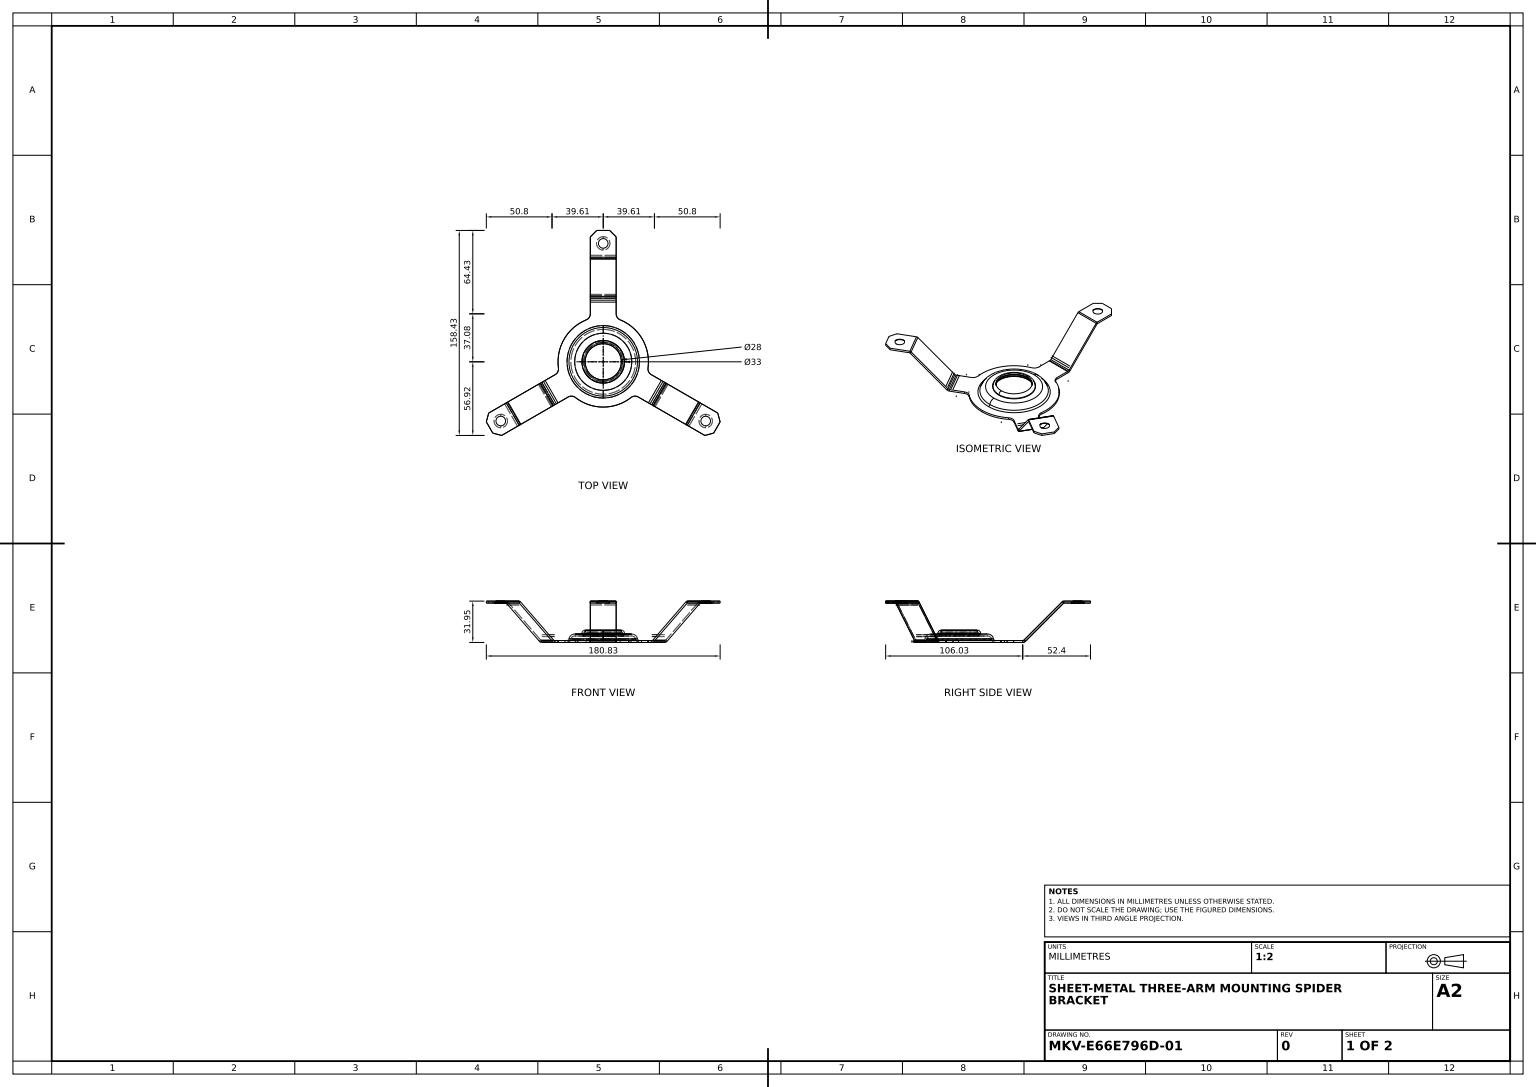
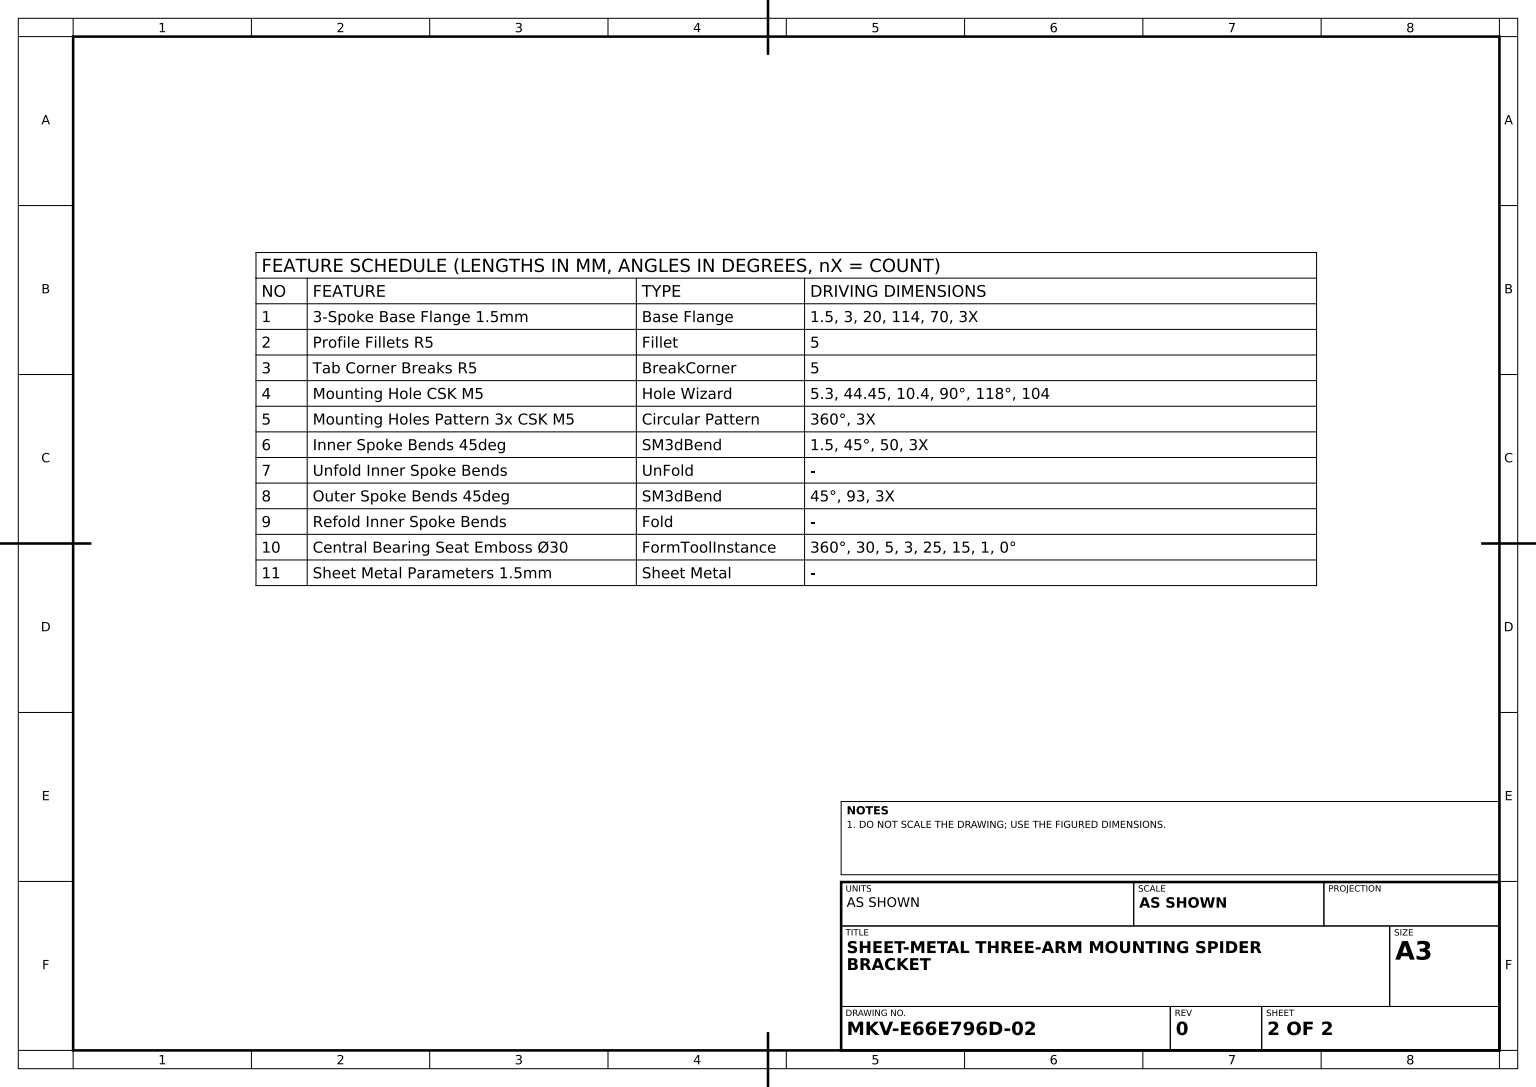
solid
v1 (-10,28.951231,-80.810298)
v2 (-10,30.011891,-79.749638)
e1 v1 v2 LINE
v3 (-10,30.451231,-80.810298)
e2 v3 v2 CIRCLE(AX(P(-10,28.951231,-80.810298),D(1,0,0),D(0,0.707106781,-0.707106781)),1.5)
e3 v1 v3 LINE
face PLANE(AX(P(-10,28.951231,-80.810298),D(1,0,0),D(0,0.707106781,-0.707106781))) rev [e1 -e2 -e3]
v4 (0,6.5,-14)
v5 (0,5.5,-15)
e4 v4 v5 CIRCLE(AX(P(0,5.5,-14),D(-1,0,0),D(0,0,1)),1)
v6 (0,5.5,15)
e5 v5 v6 CIRCLE(AX(P(0,5.5,0),D(0,-1,0),D(0,0,1)),15)
v7 (0,6.5,14)
e6 v7 v6 CIRCLE(AX(P(0,5.5,14),D(1,0,0),D(0,0,-1)),1)
e7 v7 v4 CIRCLE(AX(P(0,6.5,0),D(0,1,0),D(0,0,1)),14)
face TORUS(AX(P(0,5.5,0),D(0,-1,0),D(0,0,1)),14,1) rev [e4 e5 -e6 e7]
v8 (0,3.5,-22.08392)
v9 (0,3.5,22.08392)
e8 v8 v9 CIRCLE(AX(P(0,3.5,0),D(0,1,0),D(0,0,1)),22.08392)
v10 (0,1,25.04196)
e9 v10 v9 CIRCLE(AX(P(0,0.5,22.08392),D(-1,0,0),D(0,0,1)),3)
v11 (0,1,-25.04196)
e10 v10 v11 CIRCLE(AX(P(0,1,0),D(0,-1,0),D(0,0,-1)),25.04196)
e11 v11 v8 CIRCLE(AX(P(0,0.5,-22.08392),D(1,0,0),D(0,0,-1)),3)
face TORUS(AX(P(0,0.5,0),D(0,1,0),D(0,0,-1)),22.08392,3) rev [e8 -e9 e10 e11]
v12 (0,0,-28)
v13 (0,0,28)
e12 v12 v13 CIRCLE(AX(P(0,0,0),D(0,-1,0),D(0,0,-1)),28)
e13 v13 v12 CIRCLE(AX(P(0,0,0),D(0,-1,0),D(0,0,-1)),28)
v14 (10,0,-37.080992)
v15 (10,0,-49.116427)
e14 v14 v15 LINE
v16 (-10,0,-49.116427)
e15 v16 v15 LINE
v17 (-10,0,-37.080992)
e16 v16 v17 LINE
v18 (-13.125,0,-32.445868)
e17 v17 v18 CIRCLE(AX(P(-15,0,-37.080992),D(0,-1,0),D(0,0,1)),5)
v19 (-34.661446,0,4.856351)
e18 v18 v19 CIRCLE(AX(P(0,0,0),D(0,1,0),D(0,0,1)),35)
v20 (-37.113081,0,9.880242)
e19 v19 v20 CIRCLE(AX(P(-39.613081,0,5.550115),D(0,-1,0),D(0,0,1)),5)
v21 (-47.536074,0,15.897959)
e20 v20 v21 LINE
v22 (-37.536074,0,33.218468)
e21 v22 v21 LINE
v23 (-27.113081,0,27.20075)
e22 v22 v23 LINE
v24 (-21.536446,0,27.589518)
e23 v23 v24 CIRCLE(AX(P(-24.613081,0,31.530877),D(0,-1,0),D(0,0,1)),5)
v25 (0,0,35)
e24 v24 v25 CIRCLE(AX(P(0,0,0),D(0,1,0),D(0,0,1)),35)
v26 (21.536446,0,27.589518)
e25 v25 v26 CIRCLE(AX(P(0,0,0),D(0,1,0),D(0,0,1)),35)
v27 (27.113081,0,27.20075)
e26 v26 v27 CIRCLE(AX(P(24.613081,0,31.530877),D(0,-1,0),D(0,0,1)),5)
v28 (37.536074,0,33.218468)
e27 v27 v28 LINE
v29 (47.536074,0,15.897959)
e28 v29 v28 LINE
v30 (37.113081,0,9.880242)
e29 v29 v30 LINE
v31 (34.661446,0,4.856351)
e30 v30 v31 CIRCLE(AX(P(39.613081,0,5.550115),D(0,-1,0),D(0,0,1)),5)
v32 (13.125,0,-32.445868)
e31 v31 v32 CIRCLE(AX(P(0,0,0),D(0,1,0),D(0,0,1)),35)
e32 v32 v14 CIRCLE(AX(P(15,0,-37.080992),D(0,-1,0),D(0,0,1)),5)
face PLANE(AX(P(0,0,0),D(0,1,0),D(0,0,1))) [e12 e13] [e14 -e15 e16 e17 e18 e19 e20 -e21 e22 e23 e24 e25 e26 e27 -e28 e29 e30 e31 e32]
v33 (79.254985,28.951231,40.557887)
v34 (79.254985,28.951231,50.957887)
e33 v33 v34 CIRCLE(AX(P(79.254985,28.951231,45.757887),D(0,-1,0),D(0,0,-1)),5.2)
v35 (79.254985,30.451231,49.457887)
e34 v35 v34 LINE
v36 (79.254985,30.451231,42.057887)
e35 v35 v36 CIRCLE(AX(P(79.254985,30.451231,45.757887),D(0,1,0),D(0,0,1)),3.7)
e36 v36 v33 LINE
face CONE(AX(P(79.254985,28.951231,45.757887),D(0,-1,0),D(0,0,-1)),5.2,0.785398163) rev [e33 -e34 e35 e36]
v37 (0,1.25,26.52098)
e37 v13 v37 CIRCLE(AX(P(0,1.5,28),D(1,0,0),D(0,0,-1)),1.5)
v38 (0,1.25,-26.52098)
e38 v37 v38 CIRCLE(AX(P(0,1.25,0),D(0,-1,0),D(0,0,-1)),26.52098)
e39 v12 v38 CIRCLE(AX(P(0,1.5,-28),D(-1,0,0),D(0,0,1)),1.5)
face TORUS(AX(P(0,1.5,0),D(0,-1,0),D(0,0,1)),28,1.5) rev [-e13 e37 e38 -e39]
v39 (-10,30.451231,-96.515774)
e40 v39 v3 LINE
v40 (10,30.451231,-80.810298)
e41 v3 v40 LINE
v41 (10,30.451231,-96.515774)
e42 v40 v41 LINE
v42 (5,30.451231,-101.515774)
e43 v41 v42 LINE
v43 (-5,30.451231,-101.515774)
e44 v42 v43 LINE
e45 v43 v39 LINE
v44 (0,30.451231,-95.215774)
v45 (0,30.451231,-87.815774)
e46 v44 v45 CIRCLE(AX(P(0,30.451231,-91.515774),D(0,1,0),D(0,0,1)),3.7)
e47 v45 v44 CIRCLE(AX(P(0,30.451231,-91.515774),D(0,1,0),D(0,0,1)),3.7)
face PLANE(AX(P(0,30.451231,12.484226),D(0,1,0),D(0,0,1))) [e40 e41 e42 e43 e44 e45] [-e46 -e47]
e48 v34 v33 CIRCLE(AX(P(79.254985,28.951231,45.757887),D(0,-1,0),D(0,0,-1)),5.2)
e49 v36 v35 CIRCLE(AX(P(79.254985,30.451231,45.757887),D(0,1,0),D(0,0,1)),3.7)
face CONE(AX(P(79.254985,28.951231,45.757887),D(0,-1,0),D(0,0,-1)),5.2,0.785398163) rev [e34 e48 -e36 e49]
v46 (85.415239,30.451231,55.088014)
v47 (90.415239,30.451231,46.42776)
e50 v46 v47 LINE
v48 (85.415239,28.951231,55.088014)
e51 v46 v48 LINE
v49 (90.415239,28.951231,46.42776)
e52 v48 v49 LINE
e53 v49 v47 LINE
face PLANE(AX(P(92.915239,28.951231,42.097633),D(0.866025404,0,0.5),D(0.5,0,-0.866025404))) [-e50 e51 e52 e53]
v50 (0,5,16.5)
v51 (0,5,-16.5)
e54 v50 v51 CIRCLE(AX(P(0,5,0),D(0,1,0),D(0,0,-1)),16.5)
e55 v51 v50 CIRCLE(AX(P(0,5,0),D(0,1,0),D(0,0,-1)),16.5)
v52 (0,5,-22.08392)
v53 (0,5,22.08392)
e56 v52 v53 CIRCLE(AX(P(0,5,0),D(0,1,0),D(0,0,1)),22.08392)
e57 v53 v52 CIRCLE(AX(P(0,5,0),D(0,1,0),D(0,0,1)),22.08392)
face PLANE(AX(P(-25,5,0),D(0,-1,0),D(0,0,1))) rev [-e54 -e55] [e56 e57]
v54 (-37.536074,-1.5,33.218468)
v55 (-27.113081,-1.5,27.20075)
e58 v54 v55 LINE
e59 v55 v23 LINE
e60 v54 v22 LINE
face PLANE(AX(P(-24.047375,-1.5,25.430764),D(0.5,0,0.866025404),D(0.866025404,0,-0.5))) [e58 e59 -e22 -e60]
v56 (10,28.951231,-80.810298)
e61 v40 v56 LINE
v57 (10,28.951231,-96.515774)
e62 v56 v57 LINE
e63 v57 v41 LINE
face PLANE(AX(P(10,28.951231,-21.056794),D(1,0,0),D(0,0,-1))) [-e42 e61 e62 e63]
v58 (27.113081,-1.5,27.20075)
e64 v27 v58 LINE
v59 (37.536074,-1.5,33.218468)
e65 v58 v59 LINE
e66 v28 v59 LINE
face PLANE(AX(P(24.047375,-1.5,25.430764),D(-0.5,0,0.866025404),D(0.866025404,0,0.5))) [e64 e65 -e66 -e27]
v60 (64.983771,30.451231,49.065403)
v61 (78.585112,30.451231,56.918141)
e67 v60 v61 LINE
v62 (64.983771,28.951231,49.065403)
e68 v60 v62 LINE
v63 (78.585112,28.951231,56.918141)
e69 v62 v63 LINE
e70 v63 v61 LINE
face PLANE(AX(P(13.235718,28.951231,19.188651),D(-0.5,0,0.866025404),D(0.866025404,0,0.5))) [-e67 e68 e69 e70]
e71 v9 v8 CIRCLE(AX(P(0,3.5,0),D(0,1,0),D(0,0,1)),22.08392)
e72 v11 v10 CIRCLE(AX(P(0,1,0),D(0,-1,0),D(0,0,-1)),25.04196)
face TORUS(AX(P(0,0.5,0),D(0,1,0),D(0,0,-1)),22.08392,3) rev [e71 -e11 e72 e9]
v64 (34.661446,-1.5,4.856351)
e73 v31 v64 LINE
v65 (13.125,-1.5,-32.445868)
e74 v64 v65 CIRCLE(AX(P(0,-1.5,0),D(0,1,0),D(0,0,1)),35)
e75 v65 v32 LINE
face CYL(AX(P(0,-1.5,0),D(0,1,0),D(0,0,1)),35) [-e31 e73 e74 e75]
v66 (0,-1.5,28)
e76 v66 v10 CIRCLE(AX(P(0,1.5,28),D(1,0,0),D(0,0,-1)),3)
v67 (0,-1.5,-28)
e77 v66 v67 CIRCLE(AX(P(0,-1.5,0),D(0,-1,0),D(0,0,1)),28)
e78 v67 v11 CIRCLE(AX(P(0,1.5,-28),D(-1,0,0),D(0,0,1)),3)
face TORUS(AX(P(0,1.5,0),D(0,-1,0),D(0,0,1)),28,3) [-e10 -e76 e77 e78]
v68 (0,28.951231,-86.315774)
e79 v45 v68 LINE
v69 (0,28.951231,-96.715774)
e80 v68 v69 CIRCLE(AX(P(0,28.951231,-91.515774),D(0,-1,0),D(0,0,-1)),5.2)
e81 v44 v69 LINE
face CONE(AX(P(0,28.951231,-91.515774),D(0,-1,0),D(0,0,-1)),5.2,0.785398163) rev [e46 e79 e80 -e81]
v70 (-38.454632,0.43934,33.748798)
e82 v22 v70 CIRCLE(AX(P(-37.536074,1.5,33.218468),D(-0.5,0,-0.866025404),D(-0.866025404,0,0.5)),1.5)
v71 (-39.373191,-0.62132,34.279128)
e83 v71 v70 LINE
e84 v54 v71 CIRCLE(AX(P(-37.536074,1.5,33.218468),D(-0.5,0,-0.866025404),D(-0.866025404,0,0.5)),3)
face PLANE(AX(P(-37.536074,1.5,33.218468),D(0.5,0,0.866025404),D(0.866025404,0,-0.5))) [e60 e82 -e83 -e84]
v72 (10,-1.5,-49.116427)
e85 v15 v72 LINE
v73 (10,-1.5,-37.080992)
e86 v14 v73 LINE
e87 v73 v72 LINE
face PLANE(AX(P(10,-1.5,-33.54102),D(1,0,0),D(0,0,-1))) [-e85 -e14 e86 e87]
v74 (-64.983771,28.951231,49.065403)
v75 (-64.983771,30.451231,49.065403)
e88 v74 v75 LINE
v76 (-64.065213,30.011891,48.535073)
e89 v74 v76 LINE
e90 v75 v76 CIRCLE(AX(P(-64.983771,28.951231,49.065403),D(-0.5,0,-0.866025404),D(-0.612372436,0.707106781,0.353553391)),1.5)
face PLANE(AX(P(-64.983771,28.951231,49.065403),D(-0.5,0,-0.866025404),D(-0.612372436,0.707106781,0.353553391))) rev [-e88 e89 -e90]
v77 (47.536074,-1.5,15.897959)
e91 v77 v29 LINE
v78 (37.113081,-1.5,9.880242)
e92 v77 v78 LINE
e93 v78 v30 LINE
face PLANE(AX(P(34.047375,-1.5,8.110256),D(0.5,0,-0.866025404),D(-0.866025404,0,-0.5))) [-e91 e92 e93 -e29]
v79 (49.373191,-0.62132,16.95862)
v80 (39.373191,-0.62132,34.279128)
e94 v79 v80 LINE
e95 v80 v59 CIRCLE(AX(P(37.536074,1.5,33.218468),D(0.5,0,-0.866025404),D(-0.866025404,0,-0.5)),3)
e96 v77 v59 LINE
e97 v77 v79 CIRCLE(AX(P(47.536074,1.5,15.897959),D(-0.5,0,0.866025404),D(0.866025404,0,0.5)),3)
face CYL(AX(P(53.336404,1.5,5.851493),D(-0.5,0,0.866025404),D(0.866025404,0,0.5)),3) [e94 e95 -e96 e97]
v81 (-10,-1.5,-49.116427)
e98 v81 v16 LINE
v82 (-10,-1.5,-37.080992)
e99 v81 v82 LINE
e100 v82 v17 LINE
face PLANE(AX(P(-10,-1.5,-33.54102),D(-1,0,0),D(0,0,1))) [-e16 -e98 e99 e100]
v83 (5,28.951231,-101.515774)
v84 (-5,28.951231,-101.515774)
e101 v83 v84 LINE
e102 v84 v43 LINE
e103 v42 v83 LINE
face PLANE(AX(P(-10,28.951231,-101.515774),D(0,0,-1),D(-1,0,0))) [e101 e102 -e44 e103]
v85 (-90.415239,30.451231,46.42776)
v86 (-90.415239,28.951231,46.42776)
e104 v85 v86 LINE
v87 (-88.585112,30.451231,39.597633)
e105 v87 v85 LINE
v88 (-88.585112,28.951231,39.597633)
e106 v88 v87 LINE
e107 v86 v88 LINE
face PLANE(AX(P(-88.585112,28.951231,39.597633),D(0.965925826,0,0.258819045),D(0,1,0))) rev [-e104 -e105 -e106 -e107]
v89 (48.454632,0.43934,16.42829)
e108 v29 v89 CIRCLE(AX(P(47.536074,1.5,15.897959),D(-0.5,0,0.866025404),D(0.866025404,0,0.5)),1.5)
v90 (38.454632,0.43934,33.748798)
e109 v90 v28 CIRCLE(AX(P(37.536074,1.5,33.218468),D(0.5,0,-0.866025404),D(0.866025404,0,0.5)),1.5)
e110 v89 v90 LINE
face CYL(AX(P(53.336404,1.5,5.851493),D(-0.5,0,0.866025404),D(0.866025404,0,0.5)),1.5) rev [-e108 e28 -e109 -e110]
v91 (74.983771,28.951231,31.744895)
e111 v91 v79 LINE
e112 v79 v89 LINE
v92 (74.065213,30.011891,31.214565)
e113 v92 v89 LINE
e114 v91 v92 LINE
face PLANE(AX(P(38.753089,-12.884357,10.827101),D(0.5,0,-0.866025404),D(-0.612372436,-0.707106781,-0.353553391))) [e111 e112 -e113 -e114]
v93 (-74.983771,30.451231,31.744895)
e115 v75 v93 LINE
v94 (-74.065213,30.011891,31.214565)
e116 v76 v94 LINE
e117 v93 v94 CIRCLE(AX(P(-74.983771,28.951231,31.744895),D(-0.5,0,-0.866025404),D(-0.612372436,0.707106781,0.353553391)),1.5)
face CYL(AX(P(-74.983771,28.951231,31.744895),D(-0.5,0,-0.866025404),D(-0.612372436,0.707106781,0.353553391)),1.5) [-e115 e90 e116 -e117]
e118 v4 v7 CIRCLE(AX(P(0,6.5,0),D(0,1,0),D(0,0,1)),14)
v95 (0,8,-14)
e119 v95 v4 LINE
v96 (0,8,14)
e120 v95 v96 CIRCLE(AX(P(0,8,0),D(0,1,0),D(0,0,-1)),14)
e121 v96 v7 LINE
face CYL(AX(P(0,5.5,0),D(0,-1,0),D(0,0,-1)),14) rev [-e118 -e119 e120 e121]
e122 v67 v66 CIRCLE(AX(P(0,-1.5,0),D(0,-1,0),D(0,0,1)),28)
face TORUS(AX(P(0,1.5,0),D(0,-1,0),D(0,0,1)),28,3) [-e78 e122 e76 -e72]
e123 v38 v37 CIRCLE(AX(P(0,1.25,0),D(0,-1,0),D(0,0,-1)),26.52098)
face TORUS(AX(P(0,1.5,0),D(0,-1,0),D(0,0,1)),28,1.5) rev [-e37 -e12 e39 e123]
v97 (10,30.011891,-79.749638)
e124 v40 v97 CIRCLE(AX(P(10,28.951231,-80.810298),D(1,0,0),D(0,0.707106781,-0.707106781)),1.5)
e125 v97 v56 LINE
face PLANE(AX(P(10,28.951231,-80.810298),D(-1,0,0),D(0,-0.707106781,0.707106781))) rev [e124 e125 -e61]
e126 v73 v65 CIRCLE(AX(P(15,-1.5,-37.080992),D(0,1,0),D(0,0,1)),5)
face CYL(AX(P(15,-1.5,-37.080992),D(0,1,0),D(0,0,1)),5) rev [-e126 -e86 -e32 -e75]
face PLANE(AX(P(47.536074,1.5,15.897959),D(0.5,0,-0.866025404),D(-0.866025404,0,-0.5))) [-e97 e91 e108 -e112]
v98 (-49.373191,-0.62132,16.95862)
v99 (-74.983771,28.951231,31.744895)
e127 v98 v99 LINE
e128 v94 v99 LINE
v100 (-48.454632,0.43934,16.42829)
e129 v100 v94 LINE
e130 v100 v98 LINE
face PLANE(AX(P(-38.753089,-12.884357,10.827101),D(-0.5,0,-0.866025404),D(-0.612372436,0.707106781,0.353553391))) [e127 -e128 -e129 e130]
v101 (-79.254985,30.451231,49.457887)
v102 (-79.254985,30.451231,42.057887)
e131 v101 v102 CIRCLE(AX(P(-79.254985,30.451231,45.757887),D(0,1,0),D(0,0,1)),3.7)
v103 (-79.254985,28.951231,40.557887)
e132 v102 v103 LINE
v104 (-79.254985,28.951231,50.957887)
e133 v103 v104 CIRCLE(AX(P(-79.254985,28.951231,45.757887),D(0,-1,0),D(0,0,-1)),5.2)
e134 v101 v104 LINE
face CONE(AX(P(-79.254985,28.951231,45.757887),D(0,-1,0),D(0,0,-1)),5.2,0.785398163) rev [e131 e132 e133 -e134]
v105 (-85.415239,30.451231,55.088014)
v106 (-78.585112,30.451231,56.918141)
e135 v105 v106 LINE
e136 v106 v75 LINE
e137 v93 v87 LINE
e138 v85 v105 LINE
e139 v102 v101 CIRCLE(AX(P(-79.254985,30.451231,45.757887),D(0,1,0),D(0,0,1)),3.7)
face PLANE(AX(P(10.811657,30.451231,-6.242113),D(0,1,0),D(0,0,1))) [e135 e136 e115 e137 e105 e138] [-e131 -e139]
v107 (74.983771,30.451231,31.744895)
e140 v91 v107 LINE
v108 (88.585112,30.451231,39.597633)
e141 v108 v107 LINE
v109 (88.585112,28.951231,39.597633)
e142 v108 v109 LINE
e143 v109 v91 LINE
face PLANE(AX(P(23.235718,28.951231,1.868143),D(0.5,0,-0.866025404),D(-0.866025404,0,-0.5))) [e140 -e141 e142 e143]
e144 v99 v88 LINE
e145 v93 v99 LINE
face PLANE(AX(P(-23.235718,28.951231,1.868143),D(-0.5,0,-0.866025404),D(-0.866025404,0,0.5))) [e144 e106 -e137 e145]
v110 (0,5.5,-16.5)
e146 v95 v110 CIRCLE(AX(P(0,5.5,-14),D(-1,0,0),D(0,0,1)),2.5)
e147 v96 v95 CIRCLE(AX(P(0,8,0),D(0,1,0),D(0,0,-1)),14)
v111 (0,5.5,16.5)
e148 v96 v111 CIRCLE(AX(P(0,5.5,14),D(1,0,0),D(0,0,-1)),2.5)
e149 v110 v111 CIRCLE(AX(P(0,5.5,0),D(0,-1,0),D(0,0,1)),16.5)
face TORUS(AX(P(0,5.5,0),D(0,-1,0),D(0,0,1)),14,2.5) [-e146 -e147 e148 -e149]
v112 (21.536446,-1.5,27.589518)
e150 v58 v112 CIRCLE(AX(P(24.613081,-1.5,31.530877),D(0,1,0),D(0,0,1)),5)
e151 v112 v26 LINE
face CYL(AX(P(24.613081,-1.5,31.530877),D(0,1,0),D(0,0,1)),5) rev [-e150 -e64 -e26 -e151]
v113 (-37.113081,-1.5,9.880242)
e152 v20 v113 LINE
v114 (-47.536074,-1.5,15.897959)
e153 v113 v114 LINE
e154 v21 v114 LINE
face PLANE(AX(P(-34.047375,-1.5,8.110256),D(-0.5,0,-0.866025404),D(-0.866025404,0,0.5))) [-e20 e152 e153 -e154]
face PLANE(AX(P(-74.983771,28.951231,31.744895),D(0.5,0,0.866025404),D(0.612372436,-0.707106781,-0.353553391))) rev [-e145 e117 e128]
e155 v48 v63 LINE
e156 v61 v46 LINE
face PLANE(AX(P(78.585112,28.951231,56.918141),D(-0.258819045,0,-0.965925826),D(0,1,0))) rev [-e70 -e155 -e51 -e156]
e157 v98 v114 CIRCLE(AX(P(-47.536074,1.5,15.897959),D(0.5,0,0.866025404),D(0.866025404,0,-0.5)),3)
e158 v100 v21 CIRCLE(AX(P(-47.536074,1.5,15.897959),D(0.5,0,0.866025404),D(-0.866025404,0,0.5)),1.5)
face PLANE(AX(P(-47.536074,1.5,15.897959),D(-0.5,0,-0.866025404),D(-0.866025404,0,0.5))) [-e157 -e130 e158 e154]
e159 v47 v108 LINE
e160 v107 v60 LINE
face PLANE(AX(P(-10.811657,30.451231,-6.242113),D(0,1,0),D(0,0,1))) [e67 e156 e50 e159 e141 e160] [-e49 -e35]
v115 (64.065213,30.011891,48.535073)
e161 v92 v115 LINE
e162 v60 v115 CIRCLE(AX(P(64.983771,28.951231,49.065403),D(-0.5,0,0.866025404),D(0.612372436,0.707106781,0.353553391)),1.5)
e163 v107 v92 CIRCLE(AX(P(74.983771,28.951231,31.744895),D(-0.5,0,0.866025404),D(0.612372436,0.707106781,0.353553391)),1.5)
face CYL(AX(P(64.983771,28.951231,49.065403),D(-0.5,0,0.866025404),D(0.612372436,0.707106781,0.353553391)),1.5) [e161 -e162 -e160 e163]
e164 v50 v111 LINE
e165 v51 v110 LINE
face CYL(AX(P(0,6.5,0),D(0,1,0),D(0,0,-1)),16.5) [e149 -e164 e54 e165]
e166 v111 v110 CIRCLE(AX(P(0,5.5,0),D(0,-1,0),D(0,0,1)),16.5)
face CYL(AX(P(0,6.5,0),D(0,1,0),D(0,0,-1)),16.5) [e164 e166 -e165 e55]
v116 (-78.585112,28.951231,56.918141)
e167 v106 v116 LINE
e168 v116 v74 LINE
face PLANE(AX(P(-13.235718,28.951231,19.188651),D(0.5,0,0.866025404),D(0.866025404,0,-0.5))) [e167 e168 e88 -e136]
v117 (-10,28.951231,-96.515774)
e169 v117 v1 LINE
e170 v39 v117 LINE
face PLANE(AX(P(-10,28.951231,-21.056794),D(-1,0,0),D(0,0,1))) [e169 e3 -e40 e170]
v118 (-21.536446,-1.5,27.589518)
e171 v24 v118 LINE
v119 (0,-1.5,35)
e172 v118 v119 CIRCLE(AX(P(0,-1.5,0),D(0,1,0),D(0,0,1)),35)
e173 v119 v25 LINE
face CYL(AX(P(0,-1.5,0),D(0,1,0),D(0,0,1)),35) [-e24 e171 e172 e173]
e174 v2 v97 LINE
face CYL(AX(P(10,28.951231,-80.810298),D(1,0,0),D(0,0.707106781,-0.707106781)),1.5) [e2 e174 -e124 -e41]
v120 (0,4.5,15)
e175 v120 v6 LINE
v121 (0,4.5,-15)
e176 v121 v5 LINE
e177 v120 v121 CIRCLE(AX(P(0,4.5,0),D(0,1,0),D(0,0,1)),15)
face CYL(AX(P(0,6.5,0),D(0,1,0),D(0,0,-1)),15) rev [e175 -e5 -e176 -e177]
v122 (-10,0.43934,-50.177087)
v123 (10,0.43934,-50.177087)
e178 v122 v123 LINE
e179 v123 v97 LINE
e180 v2 v122 LINE
face PLANE(AX(P(0,-35.54078,-14.196968),D(0,0.707106781,0.707106781),D(0,-0.707106781,0.707106781))) [e178 e179 -e174 e180]
face PLANE(AX(P(74.983771,28.951231,31.744895),D(-0.5,0,0.866025404),D(0.612372436,0.707106781,0.353553391))) rev [-e163 -e140 e114]
v124 (-10,-0.62132,-51.237747)
e181 v1 v124 LINE
e182 v1 v56 LINE
v125 (10,-0.62132,-51.237747)
e183 v125 v56 LINE
e184 v124 v125 LINE
face PLANE(AX(P(0,-36.60144,-15.257628),D(0,0.707106781,0.707106781),D(0,-0.707106781,0.707106781))) rev [-e181 e182 -e183 -e184]
v126 (0,3.5,16)
v127 (0,3.5,-16)
e185 v126 v127 CIRCLE(AX(P(0,3.5,0),D(0,-1,0),D(0,0,1)),16)
e186 v127 v126 CIRCLE(AX(P(0,3.5,0),D(0,-1,0),D(0,0,1)),16)
face PLANE(AX(P(-25,3.5,0),D(0,-1,0),D(0,0,1))) [-e71 -e8] [-e185 -e186]
e187 v38 v52 CIRCLE(AX(P(0,0.5,-22.08392),D(1,0,0),D(0,0,-1)),4.5)
e188 v37 v53 CIRCLE(AX(P(0,0.5,22.08392),D(-1,0,0),D(0,0,1)),4.5)
face TORUS(AX(P(0,0.5,0),D(0,1,0),D(0,0,-1)),22.08392,4.5) [-e123 e187 -e57 -e188]
e189 v64 v78 CIRCLE(AX(P(39.613081,-1.5,5.550115),D(0,1,0),D(0,0,1)),5)
face CYL(AX(P(39.613081,-1.5,5.550115),D(0,1,0),D(0,0,1)),5) rev [-e30 -e93 -e189 -e73]
v128 (-34.661446,-1.5,4.856351)
e190 v128 v19 LINE
v129 (-13.125,-1.5,-32.445868)
e191 v18 v129 LINE
e192 v129 v128 CIRCLE(AX(P(0,-1.5,0),D(0,1,0),D(0,0,1)),35)
face CYL(AX(P(0,-1.5,0),D(0,1,0),D(0,0,1)),35) [e190 -e18 e191 e192]
e193 v113 v128 CIRCLE(AX(P(-39.613081,-1.5,5.550115),D(0,1,0),D(0,0,1)),5)
face CYL(AX(P(-39.613081,-1.5,5.550115),D(0,1,0),D(0,0,1)),5) rev [-e152 -e19 -e190 -e193]
e194 v125 v72 CIRCLE(AX(P(10,1.5,-49.116427),D(-1,0,0),D(0,0,1)),3)
e195 v81 v72 LINE
e196 v81 v124 CIRCLE(AX(P(-10,1.5,-49.116427),D(1,0,0),D(0,0,-1)),3)
face CYL(AX(P(-20.133872,1.5,-49.116427),D(1,0,0),D(0,0,-1)),3) [e194 -e195 e196 e184]
v130 (-85.415239,28.951231,55.088014)
e197 v86 v130 LINE
e198 v74 v99 LINE
e199 v116 v130 LINE
e200 v104 v103 CIRCLE(AX(P(-79.254985,28.951231,45.757887),D(0,-1,0),D(0,0,-1)),5.2)
face PLANE(AX(P(10.811657,28.951231,-6.242113),D(0,1,0),D(0,0,1))) rev [-e197 e107 -e144 -e198 -e168 e199] [-e200 -e133]
e201 v90 v80 LINE
face PLANE(AX(P(37.536074,1.5,33.218468),D(-0.5,0,0.866025404),D(0.866025404,0,0.5))) [e109 e66 -e95 -e201]
e202 v123 v125 LINE
face PLANE(AX(P(10,-12.884357,-38.97471),D(1,0,0),D(0,0.707106781,-0.707106781))) [-e125 -e179 e202 e183]
e203 v16 v122 CIRCLE(AX(P(-10,1.5,-49.116427),D(1,0,0),D(0,0,-1)),1.5)
e204 v124 v122 LINE
face PLANE(AX(P(-10,1.5,-49.116427),D(-1,0,0),D(0,0,1))) [e203 -e204 -e196 e98]
e205 v115 v62 LINE
face PLANE(AX(P(64.983771,28.951231,49.065403),D(0.5,0,-0.866025404),D(-0.612372436,-0.707106781,-0.353553391))) rev [e162 e205 -e68]
e206 v70 v100 LINE
face CYL(AX(P(-31.735743,1.5,43.264934),D(-0.5,0,-0.866025404),D(-0.866025404,0,0.5)),1.5) rev [-e158 -e206 -e82 e21]
e207 v118 v55 CIRCLE(AX(P(-24.613081,-1.5,31.530877),D(0,1,0),D(0,0,1)),5)
face CYL(AX(P(-24.613081,-1.5,31.530877),D(0,1,0),D(0,0,1)),5) rev [-e171 -e23 -e59 -e207]
e208 v6 v5 CIRCLE(AX(P(0,5.5,0),D(0,-1,0),D(0,0,1)),15)
face TORUS(AX(P(0,5.5,0),D(0,-1,0),D(0,0,1)),14,1) rev [e118 e6 e208 -e4]
e209 v109 v49 LINE
face PLANE(AX(P(90.415239,28.951231,46.42776),D(-0.965925826,0,0.258819045),D(0,1,0))) rev [-e142 -e159 -e53 -e209]
face CYL(AX(P(0,5.5,0),D(0,-1,0),D(0,0,-1)),14) rev [e119 -e7 -e121 e147]
e210 v123 v15 CIRCLE(AX(P(10,1.5,-49.116427),D(-1,0,0),D(0,0,-1)),1.5)
face PLANE(AX(P(10,1.5,-49.116427),D(1,0,0),D(0,0,-1))) [e210 e85 -e194 -e202]
face PLANE(AX(P(-10,-12.884357,-38.97471),D(-1,0,0),D(0,-0.707106781,0.707106781))) [e204 -e180 -e1 e181]
face CYL(AX(P(-20.133872,1.5,-49.116427),D(1,0,0),D(0,0,-1)),1.5) rev [-e210 -e178 -e203 e15]
e211 v54 v114 LINE
e212 v129 v82 CIRCLE(AX(P(-15,-1.5,-37.080992),D(0,1,0),D(0,0,1)),5)
e213 v119 v112 CIRCLE(AX(P(0,-1.5,0),D(0,1,0),D(0,0,1)),35)
face PLANE(AX(P(0,-1.5,0),D(0,1,0),D(0,0,1))) rev [-e172 e207 -e58 e211 -e153 e193 -e192 e212 -e99 e195 -e87 e126 -e74 e189 -e92 e96 -e65 e150 -e213] [-e77 -e122]
e214 v117 v84 LINE
e215 v83 v57 LINE
e216 v69 v68 CIRCLE(AX(P(0,28.951231,-91.515774),D(0,-1,0),D(0,0,-1)),5.2)
face PLANE(AX(P(0,28.951231,12.484226),D(0,1,0),D(0,0,1))) rev [-e182 -e169 e214 -e101 e215 -e62] [-e216 -e80]
e217 v76 v70 LINE
e218 v74 v71 LINE
face PLANE(AX(P(-28.753089,-12.884357,28.147609),D(0.5,0,0.866025404),D(0.612372436,-0.707106781,-0.353553391))) [-e217 -e89 e218 e83]
face TORUS(AX(P(0,0.5,0),D(0,1,0),D(0,0,-1)),22.08392,4.5) [-e56 -e187 -e38 e188]
e219 v91 v62 LINE
e220 v80 v62 LINE
face PLANE(AX(P(13.213493,-36.60144,7.628814),D(-0.612372436,0.707106781,-0.353553391),D(-0.126826484,0.353553391,0.926776695))) rev [-e94 -e111 e219 -e220]
e221 v130 v105 LINE
face PLANE(AX(P(-85.415239,28.951231,55.088014),D(0.258819045,0,-0.965925826),D(0,1,0))) rev [-e135 -e221 -e199 -e167]
e222 v90 v115 LINE
face PLANE(AX(P(28.753089,-12.884357,28.147609),D(-0.5,0,0.866025404),D(0.612372436,0.707106781,0.353553391))) [-e222 e201 e220 -e205]
e223 v71 v98 LINE
face PLANE(AX(P(-13.213493,-36.60144,7.628814),D(0.612372436,0.707106781,-0.353553391),D(0.126826484,0.353553391,0.926776695))) rev [-e223 -e218 e198 -e127]
face PLANE(AX(P(-5,28.951231,-101.515774),D(0.707106781,0,0.707106781),D(0,1,0))) rev [-e170 -e45 -e102 -e214]
e224 v121 v120 CIRCLE(AX(P(0,4.5,0),D(0,1,0),D(0,0,1)),15)
face CYL(AX(P(0,6.5,0),D(0,1,0),D(0,0,-1)),15) rev [-e175 -e224 e176 -e208]
e225 v126 v120 CIRCLE(AX(P(0,4.5,16),D(1,0,0),D(0,0,-1)),1)
e226 v127 v121 CIRCLE(AX(P(0,4.5,-16),D(-1,0,0),D(0,0,1)),1)
face TORUS(AX(P(0,4.5,0),D(0,-1,0),D(0,0,1)),16,1) [-e225 e185 e226 e224]
face CONE(AX(P(-79.254985,28.951231,45.757887),D(0,-1,0),D(0,0,-1)),5.2,0.785398163) rev [e200 -e132 e139 e134]
face TORUS(AX(P(0,4.5,0),D(0,-1,0),D(0,0,1)),16,1) [e225 e177 -e226 e186]
face PLANE(AX(P(12.294935,-35.54078,7.098484),D(-0.612372436,0.707106781,-0.353553391),D(-0.126826484,0.353553391,0.926776695))) [e113 e110 e222 -e161]
face CONE(AX(P(0,28.951231,-91.515774),D(0,-1,0),D(0,0,-1)),5.2,0.785398163) rev [e47 e81 e216 -e79]
face CYL(AX(P(-31.735743,1.5,43.264934),D(-0.5,0,-0.866025404),D(-0.866025404,0,0.5)),3) [-e211 e84 e223 e157]
face TORUS(AX(P(0,5.5,0),D(0,-1,0),D(0,0,1)),14,2.5) [-e148 -e120 e146 -e166]
face PLANE(AX(P(-10.811657,28.951231,-6.242113),D(0,1,0),D(0,0,1))) rev [-e48 -e33] [-e219 -e143 e209 -e52 e155 -e69]
face PLANE(AX(P(10,28.951231,-96.515774),D(-0.707106781,0,0.707106781),D(0,1,0))) rev [-e215 -e103 -e43 -e63]
face CYL(AX(P(0,-1.5,0),D(0,1,0),D(0,0,1)),35) [e151 -e25 -e173 e213]
face CYL(AX(P(-15,-1.5,-37.080992),D(0,1,0),D(0,0,1)),5) rev [-e100 -e212 -e191 -e17]
face PLANE(AX(P(-82.915239,28.951231,59.418141),D(-0.866025404,0,0.5),D(0.5,0,0.866025404))) [-e138 e104 e197 e221]
face PLANE(AX(P(-12.294935,-35.54078,7.098484),D(0.612372436,0.707106781,-0.353553391),D(0.126826484,0.353553391,0.926776695))) [e206 e129 -e116 e217]
